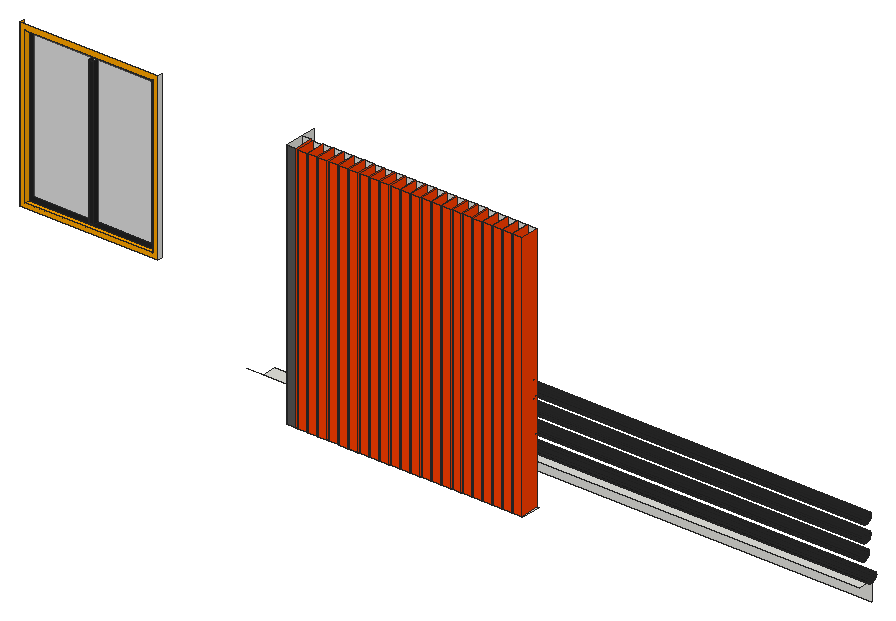
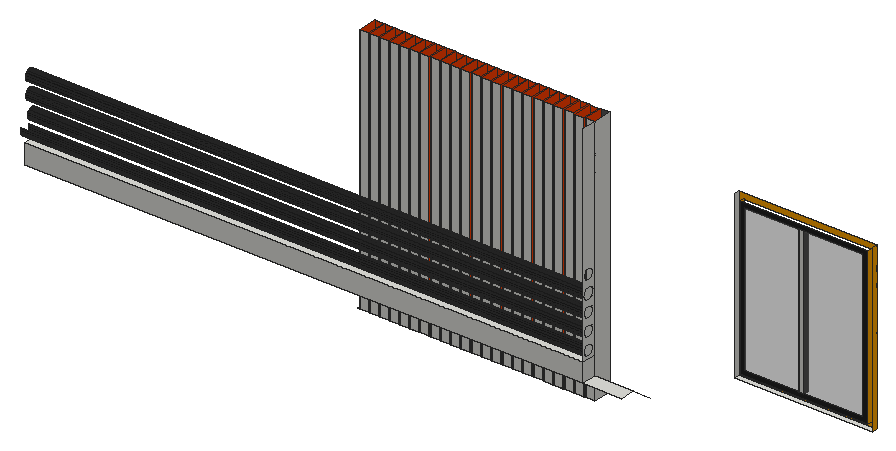
# SketchUp Ruby script. Lengths in inches.
U = 1.inch
M = Sketchup.active_model
def pt(a) = Geom::Point3d.new(a.map { |v| v * U })
def face(e, loops, mat)
  f = e.add_face(loops[0].map { |a| pt(a) })
  loops[1..].each { |l| e.add_face(l.map { |a| pt(a) }).erase! }
  f.material = f.back_material = mat if mat
  f
end
# faces: each face lists its corners as indices into pts; further lists are holes
def faces(e, pts, list, mat = nil) = list.each { |f| face(e, (f[0].is_a?(Array) ? f : [f]).map { |l| l.map { |i| pts[i] } }, mat) }
# xy, xz, yz: faces in a plane at the given z, y or x. An outline is a flat list of corners, or four numbers for a rectangle; further outlines are holes
def ring(l) = l.size == 4 ? [[l[0], l[1]], [l[2], l[1]], [l[2], l[3]], [l[0], l[3]]] : l.each_slice(2).to_a
def flat(e, list, mat, &to3) = list.each { |f| face(e, (f[0].is_a?(Array) ? f : [f]).map { |l| ring(l).map { |u, v| to3.(u, v) } }, mat) }
def xy(e, z, list, mat = nil) = flat(e, list, mat) { |x, y| [x, y, z] }
def xz(e, y, list, mat = nil) = flat(e, list, mat) { |x, z| [x, y, z] }
def yz(e, x, list, mat = nil) = flat(e, list, mat) { |y, z| [x, y, z] }
def lines(e, pts, list) = list.each { |a, b| e.add_line(pt(pts[a]), pt(pts[b])) }
# prism: a flat outline (further loops are holes) pulled along v
def prism(e, loops, v, mat = nil)
  f = face(e, loops, mat); d = Geom::Vector3d.new(v.map { |x| x * U })
  f.pushpull(f.normal.samedirection?(d) ? d.length : -d.length)
end
def box(e, o, s, mat = nil) = prism(e, [[o, [o[0] + s[0], o[1], o[2]], [o[0] + s[0], o[1] + s[1], o[2]], [o[0], o[1] + s[1], o[2]]]], [0, 0, s[2]], mat)
def at(x, y, z, deg = 0) = Geom::Transformation.translation(pt([x, y, z])) * Geom::Transformation.rotation(ORIGIN, Z_AXIS, deg.degrees)
def axes(o, x, y, z) = Geom::Transformation.new([*x, 0, *y, 0, *z, 0, *pt(o).to_a, 1])
def part(name) = M.definitions.add(name)
# library, detail: a bought-in or finely detailed component or shape, given as its bounding box
def library(name, o, s) = part(name).tap { |d| box(d.entities, o, s) }
def detail(e, o, s) = box(e.add_group.entities, o, s)
def put(e, d, t, mat = nil) = e.add_instance(d, t).tap { |i| i.material = mat if mat }
def group(e, t, mat = nil) = e.add_group.tap { |g| g.transformation = t; g.material = mat if mat }.entities
root = M.entities
M.materials.add("[0038_Orange]").color = [255, 165, 0]
M.materials.add("[0136_Charcoal]").color = [35, 35, 35]
M.materials.add("[Color B05]").color = [255, 63, 0]
M.materials.add("[Color M06]").color = [86, 86, 86]
M.materials.add("[Translucent Glass Gray]").color = [128, 128, 128]
M.materials["[Translucent Glass Gray]"].alpha = 0.5
xy(root,214.25,[[204.375,15,209.93,26.8125],[209.93,15,211.25,26.8125],[211.25,15,216.81,26.8125],[216.81,15,217.625,26.8125],[217.625,15,223.18,26.8125],
  [223.18,15,224,26.8125],[224,15,229.56,26.8125],[229.56,15,230.375,26.8125],[230.375,15,235.93,26.8125],[235.93,15,236.75,26.8125],
  [236.75,15,242.31,26.8125],[242.31,15,243.125,26.8125],[243.125,15,248.68,26.8125],[248.68,15,249.5,26.8125],[249.5,15,255.06,26.8125],
  [255.06,15,255.875,26.8125],[255.875,15,261.43,26.8125],[261.43,15,262.25,26.8125],[262.25,15,267.81,26.8125],[267.81,15,268.625,26.8125],
  [268.625,15,274.18,26.8125],[274.18,15,275,26.8125],[275,15,280.56,26.8125],[280.56,15,281.375,26.8125],[281.375,15,286.93,26.8125],
  [286.93,15,287.75,26.8125],[287.75,15,293.31,26.8125],[293.31,15,294.125,26.8125],[294.125,15,299.68,26.8125],[299.68,15,300.5,26.8125],
  [300.5,15,306.06,26.8125],[306.06,15,306.875,26.8125],[306.875,15,312.43,26.8125],[312.43,15,313.125,26.8125],[313.125,15,318.68,26.8125],
  [318.68,15,319.375,26.8125],[319.375,15,324.93,26.8125],[324.93,15,325.625,26.8125],[325.625,15,331.18,26.8125],[331.18,15,331.875,26.8125],
  [331.875,15,337.43,26.8125],[337.43,15,338.125,26.8125],[338.125,15,343.68,26.8125],[343.68,15,344.375,26.8125],[344.375,15,349.93,26.8125],
  [349.93,15,350.625,26.8125]])
xy(root,228,[[180.5,27,204.375,36]])
xy(root,240,[[204.375,26.8125,549.5625,36]])
xy(root,264.24,[[25.4,33,110.21,36]])
xy(root,267.24,[[28.4,33,107.21,36]],"[0038_Orange]")
xy(root,270,[[67.8,33,70.67,36]])
xz(root,15,[[211.25,214.25,216.81,368.4375],[217.625,214.25,223.18,368.875],[224,214.25,229.56,368.875],[230.375,214.25,235.93,368.875],[236.75,214.25,242.31,368.875],
  [243.125,214.25,248.68,368.875],[249.5,214.25,255.06,368.875],[255.875,214.25,261.43,368.875],[262.25,214.25,267.81,368.875],[268.625,214.25,274.18,368.875],
  [275,214.25,280.56,368.875],[281.375,214.25,286.93,368.875],[287.75,214.25,293.31,368.875],[294.125,214.25,299.68,368.875],[300.5,214.25,306.06,368.875],
  [306.875,214.25,312.43,368.875],[313.125,214.25,318.68,368.875],[319.375,214.25,324.93,368.6875],[325.625,214.25,331.18,368.6875],[331.875,214.25,337.43,368.6875],
  [338.125,214.25,343.68,368.6875],[344.375,214.25,349.93,368.6875]],"[Color B05]")
xz(root,15,[[204.375,214.25,209.93,368.875]],"[Color M06]")
xz(root,26.8125,[[204.375,214.25,209.93,240],[209.93,214.25,211.25,240],[211.25,214.25,216.81,240],[216.81,214.25,217.625,240],[217.625,214.25,223.18,240],
  [223.18,214.25,224,240],[224,214.25,229.56,240],[229.56,214.25,230.375,240],[230.375,214.25,235.93,240],[235.93,214.25,236.75,240],
  [236.75,214.25,242.31,240],[242.31,214.25,243.125,240],[243.125,214.25,248.68,240],[248.68,214.25,249.5,240],[249.5,214.25,255.06,240],
  [255.06,214.25,255.875,240],[255.875,214.25,261.43,240],[261.43,214.25,262.25,240],[262.25,214.25,267.81,240],[267.81,214.25,268.625,240],
  [268.625,214.25,274.18,240],[274.18,214.25,275,240],[275,214.25,280.56,240],[280.56,214.25,281.375,240],[281.375,214.25,286.93,240],
  [286.93,214.25,287.75,240],[287.75,214.25,293.31,240],[293.31,214.25,294.125,240],[294.125,214.25,299.68,240],[299.68,214.25,300.5,240],
  [300.5,214.25,306.06,240],[306.06,214.25,306.875,240],[306.875,214.25,312.43,240],[312.43,214.25,313.125,240],[313.125,214.25,318.68,240],
  [318.68,214.25,319.375,240],[319.375,214.25,324.93,240],[324.93,214.25,325.625,240],[325.625,214.25,331.18,240],[331.18,214.25,331.875,240],
  [331.875,214.25,337.43,240],[337.43,214.25,338.125,240],[338.125,214.25,343.68,240],[343.68,214.25,344.375,240],[344.375,214.25,349.93,240],
  [204.375,240,209.93,368.875],[211.25,240,216.81,368.4375],[217.625,240,223.18,368.875],[224,240,229.56,368.875],[230.375,240,235.93,368.875],
  [236.75,240,242.31,368.875],[243.125,240,248.68,368.875],[249.5,240,255.06,368.875],[255.875,240,261.43,368.875],[262.25,240,267.81,368.875],
  [268.625,240,274.18,368.875],[275,240,280.56,368.875],[281.375,240,286.93,368.875],[287.75,240,293.31,368.875],[294.125,240,299.68,368.875],
  [300.5,240,306.06,368.875],[306.875,240,312.43,368.875],[313.125,240,318.68,368.875],[319.375,240,324.93,368.6875],[325.625,240,331.18,368.6875],
  [331.875,240,337.43,368.6875],[338.125,240,343.68,368.6875],[344.375,240,349.93,368.6875]])
xz(root,33,[[[25.4,264.24,110.21,366.11],[28.4,267.24,107.21,363.11]]],"[0038_Orange]")
xz(root,33,[[67.8,270,70.67,360.35]],"[0136_Charcoal]")
xz(root,36,[[204.375,228,549.5625,240],[67.8,270,70.67,360.35]])
xz(root,36,[[[28.4,267.24,107.21,363.11],[31.16,270,104.45,360.35]]],"[0136_Charcoal]")
xz(root,36,[[31.16,270,67.8,360.35],[70.67,270,104.45,360.35]],"[Translucent Glass Gray]")
yz(root,25.4,[[33,264.24,36,366.11]],"[0038_Orange]")
yz(root,28.4,[[33,267.24,36,363.11]],"[0038_Orange]")
yz(root,67.8,[[33,270,36,360.35]],"[0136_Charcoal]")
yz(root,70.67,[[33,270,36,360.35]],"[0136_Charcoal]")
yz(root,107.21,[[33,267.24,36,363.11]],"[0038_Orange]")
yz(root,110.21,[[33,264.24,36,366.11]])
yz(root,204.375,[[15,214.25,26.8125,368.875],[26.8125,216.1875,27,228],[26.8125,228,27,240],[27,228,36,240],[[26.8125,240,36,368.875],[31.79,262.25,30.91,262.36,30.1,262.7,29.4,263.23,28.86,263.93,28.53,264.75,28.41,265.62,28.53,266.49,28.86,267.31,29.4,268.01,30.1,268.54,30.91,268.88,31.79,269,32.66,268.88,33.47,268.54,34.17,268.01,34.71,267.31,35.05,266.49,35.16,265.62,35.05,264.75,34.71,263.93,34.17,263.23,33.47,262.7,32.66,262.36],[31.79,272.75,30.91,272.86,30.1,273.2,29.4,273.73,28.86,274.43,28.53,275.25,28.41,276.12,28.53,276.99,28.86,277.81,29.4,278.51,30.1,279.04,30.91,279.38,31.79,279.5,32.66,279.38,33.47,279.04,34.17,278.51,34.71,277.81,35.05,276.99,35.16,276.12,35.05,275.25,34.71,274.43,34.17,273.73,33.47,273.2,32.66,272.86],[31.79,283.25,30.91,283.36,30.1,283.7,29.4,284.23,28.86,284.93,28.53,285.75,28.41,286.62,28.53,287.49,28.86,288.31,29.4,289.01,30.1,289.54,30.91,289.88,31.79,290,32.66,289.88,33.47,289.54,34.17,289.01,34.71,288.31,35.05,287.49,35.16,286.62,35.05,285.75,34.71,284.93,34.17,284.23,33.47,283.7,32.66,283.36],[31.79,241.25,30.91,241.36,30.1,241.7,29.4,242.23,28.86,242.93,28.53,243.75,28.41,244.62,28.53,245.49,28.86,246.31,29.4,247.01,30.1,247.54,30.91,247.88,31.79,248,32.66,247.88,33.47,247.54,34.17,247.01,34.71,246.31,35.05,245.49,35.16,244.62,35.05,243.75,34.71,242.93,34.17,242.23,33.47,241.7,32.66,241.36],[31.79,251.75,30.91,251.86,30.1,252.2,29.4,252.73,28.86,253.43,28.53,254.25,28.41,255.12,28.53,255.99,28.86,256.81,29.4,257.51,30.1,258.04,30.91,258.38,31.79,258.5,32.66,258.38,33.47,258.04,34.17,257.51,34.71,256.81,35.05,255.99,35.16,255.12,35.05,254.25,34.71,253.43,34.17,252.73,33.47,252.2,32.66,251.86]],
  [31.79,241.25,30.91,241.36,30.1,241.7,29.4,242.23,28.86,242.93,28.53,243.75,28.41,244.62,28.53,245.49,28.86,246.31,29.4,247.01,30.1,247.54,30.91,247.88,31.79,248,32.66,247.88,33.47,247.54,34.17,247.01,34.71,246.31,35.05,245.49,35.16,244.62,35.05,243.75,34.71,242.93,34.17,242.23,33.47,241.7,32.66,241.36],[31.79,251.75,30.91,251.86,30.1,252.2,29.4,252.73,28.86,253.43,28.53,254.25,28.41,255.12,28.53,255.99,28.86,256.81,29.4,257.51,30.1,258.04,30.91,258.38,31.79,258.5,32.66,258.38,33.47,258.04,34.17,257.51,34.71,256.81,35.05,255.99,35.16,255.12,35.05,254.25,34.71,253.43,34.17,252.73,33.47,252.2,32.66,251.86],[31.79,262.25,30.91,262.36,30.1,262.7,29.4,263.23,28.86,263.93,28.53,264.75,28.41,265.62,28.53,266.49,28.86,267.31,29.4,268.01,30.1,268.54,30.91,268.88,31.79,269,32.66,268.88,33.47,268.54,34.17,268.01,34.71,267.31,35.05,266.49,35.16,265.62,35.05,264.75,34.71,263.93,34.17,263.23,33.47,262.7,32.66,262.36],[31.79,272.75,30.91,272.86,30.1,273.2,29.4,273.73,28.86,274.43,28.53,275.25,28.41,276.12,28.53,276.99,28.86,277.81,29.4,278.51,30.1,279.04,30.91,279.38,31.79,279.5,32.66,279.38,33.47,279.04,34.17,278.51,34.71,277.81,35.05,276.99,35.16,276.12,35.05,275.25,34.71,274.43,34.17,273.73,33.47,273.2,32.66,272.86]])
yz(root,209.93,[[15,214.25,26.8125,368.875]],"[Color B05]")
yz(root,211.25,[[15,214.25,26.8125,368.4375]],"[Color B05]")
yz(root,216.81,[[15,214.25,26.8125,368.4375]],"[Color B05]")
yz(root,217.625,[[15,214.25,26.8125,368.875]],"[Color B05]")
yz(root,223.18,[[15,214.25,26.8125,368.875]],"[Color B05]")
yz(root,224,[[15,214.25,26.8125,368.875]],"[Color B05]")
yz(root,229.56,[[15,214.25,26.8125,368.875]],"[Color B05]")
yz(root,230.375,[[15,214.25,26.8125,368.875]],"[Color B05]")
yz(root,235.93,[[15,214.25,26.8125,368.875]],"[Color B05]")
yz(root,236.75,[[15,214.25,26.8125,368.875]],"[Color B05]")
yz(root,242.31,[[15,214.25,26.8125,368.875]],"[Color B05]")
yz(root,243.125,[[15,214.25,26.8125,368.875]],"[Color B05]")
yz(root,248.68,[[15,214.25,26.8125,368.875]],"[Color B05]")
yz(root,249.5,[[15,214.25,26.8125,368.875]],"[Color B05]")
yz(root,255.06,[[15,214.25,26.8125,368.875]],"[Color B05]")
yz(root,255.875,[[15,214.25,26.8125,368.875]],"[Color B05]")
yz(root,261.43,[[15,214.25,26.8125,368.875]],"[Color B05]")
yz(root,262.25,[[15,214.25,26.8125,368.875]],"[Color B05]")
yz(root,267.81,[[15,214.25,26.8125,368.875]],"[Color B05]")
yz(root,268.625,[[15,214.25,26.8125,368.875]],"[Color B05]")
yz(root,274.18,[[15,214.25,26.8125,368.875]],"[Color B05]")
yz(root,275,[[15,214.25,26.8125,368.875]],"[Color B05]")
yz(root,280.56,[[15,214.25,26.8125,368.875]],"[Color B05]")
yz(root,281.375,[[15,214.25,26.8125,368.875]],"[Color B05]")
yz(root,286.93,[[15,214.25,26.8125,368.875]],"[Color B05]")
yz(root,287.75,[[15,214.25,26.8125,368.875]],"[Color B05]")
yz(root,293.31,[[15,214.25,26.8125,368.875]],"[Color B05]")
yz(root,294.125,[[15,214.25,26.8125,368.875]],"[Color B05]")
yz(root,299.68,[[15,214.25,26.8125,368.875]],"[Color B05]")
yz(root,300.5,[[15,214.25,26.8125,368.875]],"[Color B05]")
yz(root,306.06,[[15,214.25,26.8125,368.875]],"[Color B05]")
yz(root,306.875,[[15,214.25,26.8125,368.875]],"[Color B05]")
yz(root,312.43,[[15,214.25,26.8125,368.875]],"[Color B05]")
yz(root,313.125,[[15,214.25,26.8125,368.875]],"[Color B05]")
yz(root,318.68,[[15,214.25,26.8125,368.875]],"[Color B05]")
yz(root,319.375,[[15,214.25,26.8125,368.6875]],"[Color B05]")
yz(root,324.93,[[15,214.25,26.8125,368.6875]],"[Color B05]")
yz(root,325.625,[[15,214.25,26.8125,368.6875]],"[Color B05]")
yz(root,331.18,[[15,214.25,26.8125,368.6875]],"[Color B05]")
yz(root,331.875,[[15,214.25,26.8125,368.6875]],"[Color B05]")
yz(root,337.43,[[15,214.25,26.8125,368.6875]],"[Color B05]")
yz(root,338.125,[[15,214.25,26.8125,368.6875]],"[Color B05]")
yz(root,343.68,[[15,214.25,26.8125,368.6875]],"[Color B05]")
yz(root,344.375,[[15,214.25,26.8125,368.6875]],"[Color B05]")
yz(root,349.93,[[15,214.25,26.8125,368.6875]],"[Color B05]")
p = [[204.375,30.91,241.36],[204.375,31.79,241.25],[552.875,31.79,241.25],[552.875,30.91,241.36],[204.375,32.66,241.36],[552.875,32.66,241.36],
  [204.375,30.1,241.7],[552.875,30.1,241.7],[204.375,33.47,241.7],[552.875,33.47,241.7],[204.375,29.4,242.23],[552.875,29.4,242.23],
  [204.375,34.17,242.23],[552.875,34.17,242.23],[204.375,28.86,242.93],[552.875,28.86,242.93],[204.375,34.71,242.93],[552.875,34.71,242.93],
  [204.375,28.53,243.75],[552.875,28.53,243.75],[204.375,35.05,243.75],[552.875,35.05,243.75],[204.375,28.41,244.62],[552.875,28.41,244.62],
  [204.375,35.16,244.62],[552.875,35.16,244.62],[204.375,28.53,245.49],[552.875,28.53,245.49],[204.375,35.05,245.49],[552.875,35.05,245.49],
  [204.375,28.86,246.31],[552.875,28.86,246.31],[204.375,34.71,246.31],[552.875,34.71,246.31],[204.375,30.91,251.86],[204.375,31.79,251.75],
  [548.3125,31.79,251.75],[548.3125,30.91,251.86],[204.375,32.66,251.86],[548.3125,32.66,251.86],[204.375,30.1,252.2],[548.3125,30.1,252.2],
  [204.375,33.47,252.2],[548.3125,33.47,252.2],[204.375,29.4,252.73],[548.3125,29.4,252.73],[204.375,34.17,252.73],[548.3125,34.17,252.73],
  [204.375,28.86,253.43],[548.3125,28.86,253.43],[204.375,34.71,253.43],[548.3125,34.71,253.43],[204.375,28.53,254.25],[548.3125,28.53,254.25],
  [204.375,35.05,254.25],[548.3125,35.05,254.25],[204.375,28.41,255.12],[548.3125,28.41,255.12],[204.375,35.16,255.12],[548.3125,35.16,255.12],
  [204.375,28.53,255.99],[548.3125,28.53,255.99],[204.375,35.05,255.99],[548.3125,35.05,255.99],[204.375,28.86,256.81],[548.3125,28.86,256.81],
  [204.375,34.71,256.81],[548.3125,34.71,256.81],[204.375,29.4,257.51],[548.3125,29.4,257.51],[204.375,34.17,257.51],[548.3125,34.17,257.51],
  [204.375,30.1,258.04],[548.3125,30.1,258.04],[204.375,33.47,258.04],[548.3125,33.47,258.04],[204.375,30.91,258.38],[548.3125,30.91,258.38],
  [204.375,32.66,258.38],[548.3125,32.66,258.38],[204.375,31.79,258.5],[548.3125,31.79,258.5],[204.375,30.91,262.36],[204.375,31.79,262.25],
  [549.4375,31.79,262.25],[549.4375,30.91,262.36],[204.375,32.66,262.36],[549.4375,32.66,262.36],[204.375,30.1,262.7],[549.4375,30.1,262.7],
  [204.375,33.47,262.7],[549.4375,33.47,262.7],[204.375,29.4,263.23],[549.4375,29.4,263.23],[204.375,34.17,263.23],[549.4375,34.17,263.23],
  [204.375,28.86,263.93],[549.4375,28.86,263.93],[204.375,34.71,263.93],[549.4375,34.71,263.93],[204.375,28.53,264.75],[549.4375,28.53,264.75],
  [204.375,35.05,264.75],[549.4375,35.05,264.75],[204.375,28.41,265.62],[549.4375,28.41,265.62],[204.375,35.16,265.62],[549.4375,35.16,265.62],
  [204.375,28.53,266.49],[549.4375,28.53,266.49],[204.375,35.05,266.49],[549.4375,35.05,266.49],[204.375,28.86,267.31],[549.4375,28.86,267.31],
  [204.375,34.71,267.31],[549.4375,34.71,267.31],[204.375,29.4,268.01],[549.4375,29.4,268.01],[204.375,34.17,268.01],[549.4375,34.17,268.01],
  [204.375,30.1,268.54],[549.4375,30.1,268.54],[204.375,33.47,268.54],[549.4375,33.47,268.54],[204.375,30.91,268.88],[549.4375,30.91,268.88],
  [204.375,32.66,268.88],[549.4375,32.66,268.88],[204.375,31.79,269],[549.4375,31.79,269],[204.375,30.91,272.86],[204.375,31.79,272.75],
  [549.5625,31.79,272.75],[549.5625,30.91,272.86],[204.375,32.66,272.86],[549.5625,32.66,272.86],[204.375,30.1,273.2],[549.5625,30.1,273.2],
  [204.375,33.47,273.2],[549.5625,33.47,273.2],[204.375,29.4,273.73],[549.5625,29.4,273.73],[204.375,34.17,273.73],[549.5625,34.17,273.73],
  [204.375,28.86,274.43],[549.5625,28.86,274.43],[204.375,34.71,274.43],[549.5625,34.71,274.43],[204.375,28.53,275.25],[549.5625,28.53,275.25],
  [204.375,35.05,275.25],[549.5625,35.05,275.25],[204.375,28.41,276.12],[549.5625,28.41,276.12],[204.375,35.16,276.12],[549.5625,35.16,276.12],
  [204.375,28.53,276.99],[549.5625,28.53,276.99],[204.375,35.05,276.99],[549.5625,35.05,276.99],[204.375,28.86,277.81],[549.5625,28.86,277.81],
  [204.375,34.71,277.81],[549.5625,34.71,277.81],[204.375,29.4,278.51],[549.5625,29.4,278.51],[204.375,34.17,278.51],[549.5625,34.17,278.51],
  [204.375,30.1,279.04],[549.5625,30.1,279.04],[204.375,33.47,279.04],[549.5625,33.47,279.04],[204.375,30.91,279.38],[549.5625,30.91,279.38],
  [204.375,32.66,279.38],[549.5625,32.66,279.38],[204.375,31.79,279.5],[549.5625,31.79,279.5],[180.5,27,228],[169.75,27,228]]
faces(root,p,[[0,1,2,3],[1,4,5,2],[6,0,3,7],[4,8,9,5],[10,6,7,11],[8,12,13,9],[14,10,11,15],[12,16,17,13],
  [18,14,15,19],[16,20,21,17],[22,18,19,23],[20,24,25,21],[26,22,23,27],[24,28,29,25],[30,26,27,31],[28,32,33,29],
  [34,35,36,37],[35,38,39,36],[40,34,37,41],[38,42,43,39],[44,40,41,45],[42,46,47,43],[48,44,45,49],[46,50,51,47],
  [52,48,49,53],[50,54,55,51],[56,52,53,57],[54,58,59,55],[60,56,57,61],[58,62,63,59],[64,60,61,65],[62,66,67,63],
  [68,64,65,69],[66,70,71,67],[72,68,69,73],[70,74,75,71],[76,72,73,77],[74,78,79,75],[80,76,77,81],[78,80,81,79],
  [82,83,84,85],[83,86,87,84],[88,82,85,89],[86,90,91,87],[92,88,89,93],[90,94,95,91],[96,92,93,97],[94,98,99,95],
  [100,96,97,101],[98,102,103,99],[104,100,101,105],[102,106,107,103],[108,104,105,109],[106,110,111,107],[112,108,109,113],[110,114,115,111],
  [116,112,113,117],[114,118,119,115],[120,116,117,121],[118,122,123,119],[124,120,121,125],[122,126,127,123],[128,124,125,129],[126,128,129,127],
  [130,131,132,133],[131,134,135,132],[136,130,133,137],[134,138,139,135],[140,136,137,141],[138,142,143,139],[144,140,141,145],[142,146,147,143],
  [148,144,145,149],[146,150,151,147],[152,148,149,153],[150,154,155,151],[156,152,153,157],[154,158,159,155],[160,156,157,161],[158,162,163,159],
  [164,160,161,165],[162,166,167,163],[168,164,165,169],[166,170,171,167],[172,168,169,173],[170,174,175,171],[176,172,173,177],[174,176,177,175]],"[0136_Charcoal]")
lines(root,p,[[178,179]])
